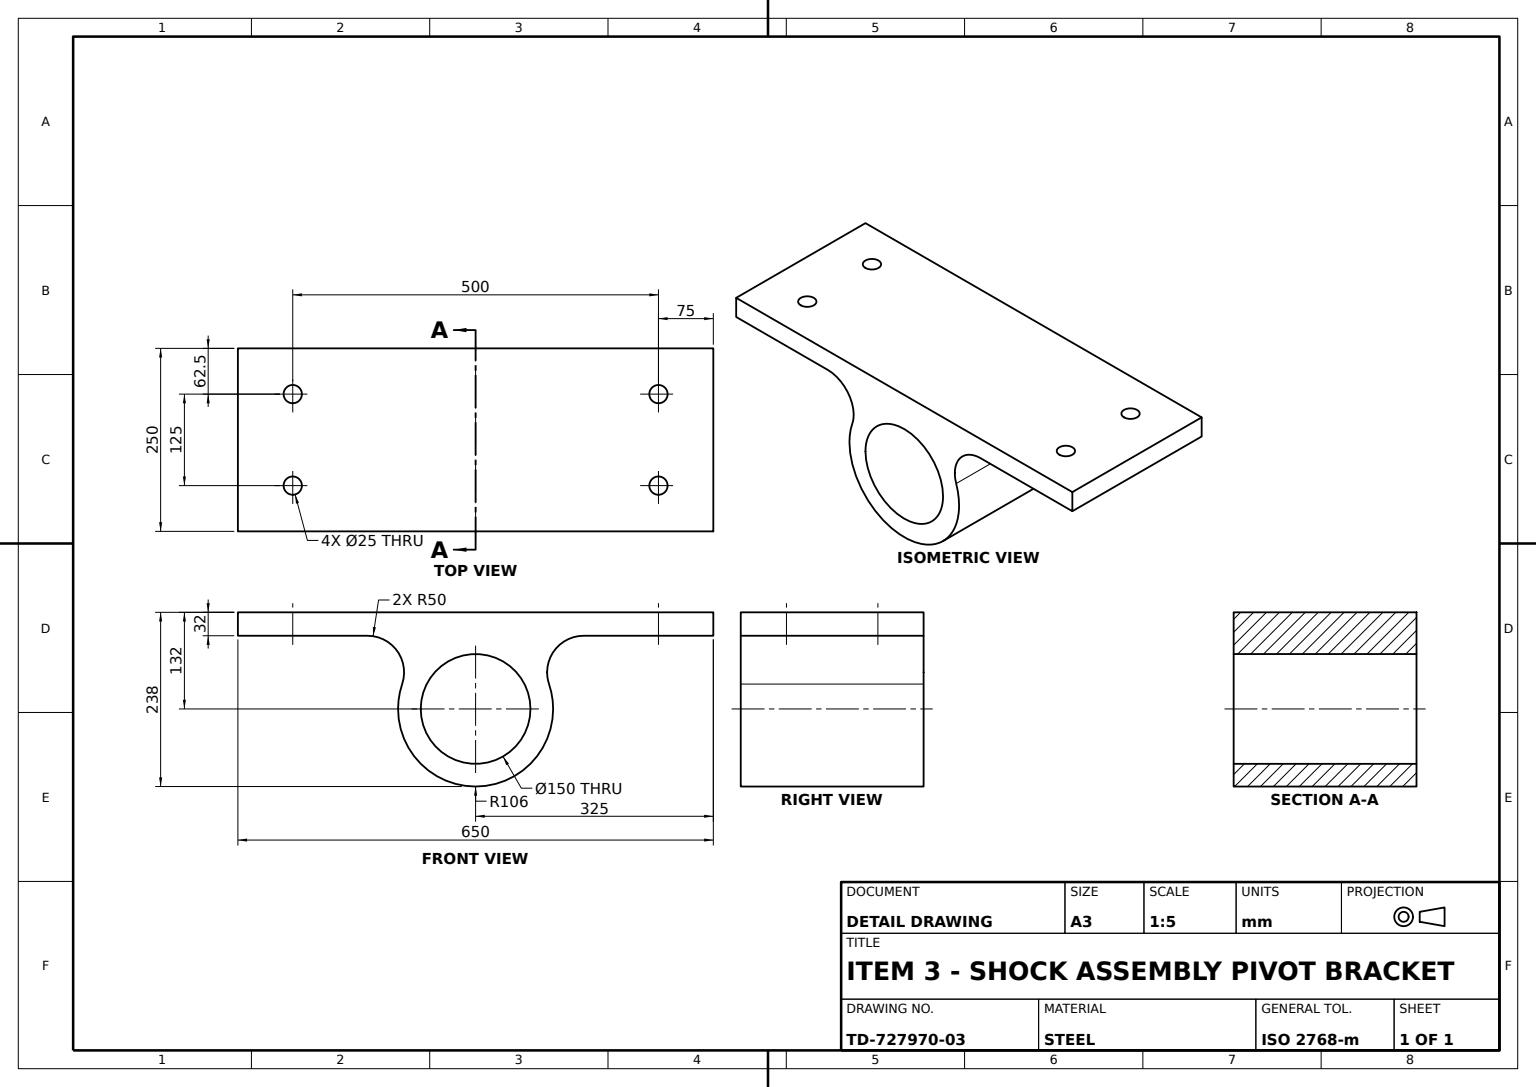
ISO-10303-21;
HEADER;
FILE_DESCRIPTION((''),'2;1');
FILE_NAME('','',(''),(''),'','','');
FILE_SCHEMA(('AUTOMOTIVE_DESIGN'));
ENDSEC;
DATA;
#1=APPLICATION_CONTEXT('');
#2=PRODUCT_CONTEXT('',#1,'mechanical');
#3=PRODUCT('','','',(#2));
#4=PRODUCT_DEFINITION_FORMATION('','',#3);
#5=PRODUCT_DEFINITION_CONTEXT('',#1,'design');
#6=PRODUCT_DEFINITION('','',#4,#5);
#7=PRODUCT_DEFINITION_SHAPE('','',#6);
#8=(LENGTH_UNIT()NAMED_UNIT(*)SI_UNIT(.MILLI.,.METRE.));
#9=(NAMED_UNIT(*)PLANE_ANGLE_UNIT()SI_UNIT($,.RADIAN.));
#10=(NAMED_UNIT(*)SI_UNIT($,.STERADIAN.)SOLID_ANGLE_UNIT());
#11=UNCERTAINTY_MEASURE_WITH_UNIT(LENGTH_MEASURE(1.E-05),#8,'distance_accuracy_value','');
#12=(GEOMETRIC_REPRESENTATION_CONTEXT(3)GLOBAL_UNCERTAINTY_ASSIGNED_CONTEXT((#11))GLOBAL_UNIT_ASSIGNED_CONTEXT((#8,#9,#10))REPRESENTATION_CONTEXT('',''));
#13=CARTESIAN_POINT('',(-250.,132.,75.));
#14=VERTEX_POINT('',#13);
#15=CARTESIAN_POINT('',(-250.,132.,50.));
#16=VERTEX_POINT('',#15);
#17=CARTESIAN_POINT('',(-250.,132.,62.5));
#18=DIRECTION('',(0.,-1.,0.));
#19=DIRECTION('',(0.,0.,-1.));
#20=AXIS2_PLACEMENT_3D('',#17,#18,#19);
#21=CIRCLE('',#20,12.5);
#22=EDGE_CURVE('',#14,#16,#21,.T.);
#23=ORIENTED_EDGE('',*,*,#22,.F.);
#24=CARTESIAN_POINT('',(-250.,100.,75.));
#25=VERTEX_POINT('',#24);
#26=CARTESIAN_POINT('',(-250.,7.,75.));
#27=DIRECTION('',(0.,1.,0.));
#28=VECTOR('',#27,1000.);
#29=LINE('',#26,#28);
#30=EDGE_CURVE('',#25,#14,#29,.T.);
#31=ORIENTED_EDGE('',*,*,#30,.F.);
#32=CARTESIAN_POINT('',(-250.,100.,50.));
#33=VERTEX_POINT('',#32);
#34=CARTESIAN_POINT('',(-250.,100.,62.5));
#35=DIRECTION('',(0.,0.,1.));
#36=AXIS2_PLACEMENT_3D('',#34,#27,#35);
#37=CIRCLE('',#36,12.5);
#38=EDGE_CURVE('',#33,#25,#37,.T.);
#39=ORIENTED_EDGE('',*,*,#38,.F.);
#40=CARTESIAN_POINT('',(-250.,7.,50.));
#41=LINE('',#40,#28);
#42=EDGE_CURVE('',#33,#16,#41,.T.);
#43=ORIENTED_EDGE('',*,*,#42,.T.);
#44=EDGE_LOOP('',(#23,#31,#39,#43));
#45=FACE_OUTER_BOUND('',#44,.T.);
#46=CARTESIAN_POINT('',(-250.,7.,62.5));
#47=AXIS2_PLACEMENT_3D('',#46,#27,#35);
#48=CYLINDRICAL_SURFACE('',#47,12.5);
#49=ADVANCED_FACE('',(#45),#48,.F.);
#50=CARTESIAN_POINT('',(-250.,100.,-75.));
#51=VERTEX_POINT('',#50);
#52=CARTESIAN_POINT('',(-250.,100.,-50.));
#53=VERTEX_POINT('',#52);
#54=CARTESIAN_POINT('',(-250.,100.,-62.5));
#55=AXIS2_PLACEMENT_3D('',#54,#27,#35);
#56=CIRCLE('',#55,12.5);
#57=EDGE_CURVE('',#51,#53,#56,.T.);
#58=ORIENTED_EDGE('',*,*,#57,.T.);
#59=EDGE_CURVE('',#53,#51,#56,.T.);
#60=ORIENTED_EDGE('',*,*,#59,.T.);
#61=EDGE_LOOP('',(#58,#60));
#62=FACE_BOUND('',#61,.T.);
#63=EDGE_CURVE('',#25,#33,#37,.T.);
#64=ORIENTED_EDGE('',*,*,#63,.T.);
#65=ORIENTED_EDGE('',*,*,#38,.T.);
#66=EDGE_LOOP('',(#64,#65));
#67=FACE_BOUND('',#66,.T.);
#68=CARTESIAN_POINT('',(-325.,100.,125.));
#69=VERTEX_POINT('',#68);
#70=CARTESIAN_POINT('',(-147.770092,100.,125.));
#71=VERTEX_POINT('',#70);
#72=DIRECTION('',(1.,0.,0.));
#73=VECTOR('',#72,1000.);
#74=LINE('',#68,#73);
#75=EDGE_CURVE('',#69,#71,#74,.T.);
#76=ORIENTED_EDGE('',*,*,#75,.F.);
#77=CARTESIAN_POINT('',(-325.,100.,-125.));
#78=VERTEX_POINT('',#77);
#79=VECTOR('',#19,1000.);
#80=LINE('',#68,#79);
#81=EDGE_CURVE('',#69,#78,#80,.T.);
#82=ORIENTED_EDGE('',*,*,#81,.T.);
#83=CARTESIAN_POINT('',(-147.770092,100.,-125.));
#84=VERTEX_POINT('',#83);
#85=LINE('',#77,#73);
#86=EDGE_CURVE('',#78,#84,#85,.T.);
#87=ORIENTED_EDGE('',*,*,#86,.T.);
#88=LINE('',#70,#79);
#89=EDGE_CURVE('',#71,#84,#88,.T.);
#90=ORIENTED_EDGE('',*,*,#89,.F.);
#91=EDGE_LOOP('',(#76,#82,#87,#90));
#92=FACE_OUTER_BOUND('',#91,.T.);
#93=AXIS2_PLACEMENT_3D('',#68,#27,#35);
#94=PLANE('',#93);
#95=ADVANCED_FACE('',(#62,#67,#92),#94,.F.);
#96=CARTESIAN_POINT('',(250.,100.,-75.));
#97=VERTEX_POINT('',#96);
#98=CARTESIAN_POINT('',(250.,100.,-50.));
#99=VERTEX_POINT('',#98);
#100=CARTESIAN_POINT('',(250.,100.,-62.5));
#101=AXIS2_PLACEMENT_3D('',#100,#27,#35);
#102=CIRCLE('',#101,12.5);
#103=EDGE_CURVE('',#97,#99,#102,.T.);
#104=ORIENTED_EDGE('',*,*,#103,.T.);
#105=EDGE_CURVE('',#99,#97,#102,.T.);
#106=ORIENTED_EDGE('',*,*,#105,.T.);
#107=EDGE_LOOP('',(#104,#106));
#108=FACE_BOUND('',#107,.T.);
#109=CARTESIAN_POINT('',(325.,100.,125.));
#110=VERTEX_POINT('',#109);
#111=CARTESIAN_POINT('',(325.,100.,-125.));
#112=VERTEX_POINT('',#111);
#113=LINE('',#109,#79);
#114=EDGE_CURVE('',#110,#112,#113,.T.);
#115=ORIENTED_EDGE('',*,*,#114,.F.);
#116=CARTESIAN_POINT('',(147.770092,100.,125.));
#117=VERTEX_POINT('',#116);
#118=LINE('',#116,#73);
#119=EDGE_CURVE('',#117,#110,#118,.T.);
#120=ORIENTED_EDGE('',*,*,#119,.F.);
#121=CARTESIAN_POINT('',(147.770092,100.,-125.));
#122=VERTEX_POINT('',#121);
#123=LINE('',#116,#79);
#124=EDGE_CURVE('',#117,#122,#123,.T.);
#125=ORIENTED_EDGE('',*,*,#124,.T.);
#126=LINE('',#121,#73);
#127=EDGE_CURVE('',#122,#112,#126,.T.);
#128=ORIENTED_EDGE('',*,*,#127,.T.);
#129=EDGE_LOOP('',(#115,#120,#125,#128));
#130=FACE_OUTER_BOUND('',#129,.T.);
#131=CARTESIAN_POINT('',(250.,100.,75.));
#132=VERTEX_POINT('',#131);
#133=CARTESIAN_POINT('',(250.,100.,50.));
#134=VERTEX_POINT('',#133);
#135=CARTESIAN_POINT('',(250.,100.,62.5));
#136=AXIS2_PLACEMENT_3D('',#135,#27,#35);
#137=CIRCLE('',#136,12.5);
#138=EDGE_CURVE('',#132,#134,#137,.T.);
#139=ORIENTED_EDGE('',*,*,#138,.T.);
#140=EDGE_CURVE('',#134,#132,#137,.T.);
#141=ORIENTED_EDGE('',*,*,#140,.T.);
#142=EDGE_LOOP('',(#139,#141));
#143=FACE_BOUND('',#142,.T.);
#144=AXIS2_PLACEMENT_3D('',#116,#27,#35);
#145=PLANE('',#144);
#146=ADVANCED_FACE('',(#108,#130,#143),#145,.F.);
#147=ORIENTED_EDGE('',*,*,#138,.F.);
#148=CARTESIAN_POINT('',(250.,132.,75.));
#149=VERTEX_POINT('',#148);
#150=CARTESIAN_POINT('',(250.,7.,75.));
#151=LINE('',#150,#28);
#152=EDGE_CURVE('',#132,#149,#151,.T.);
#153=ORIENTED_EDGE('',*,*,#152,.T.);
#154=CARTESIAN_POINT('',(250.,132.,50.));
#155=VERTEX_POINT('',#154);
#156=CARTESIAN_POINT('',(250.,132.,62.5));
#157=AXIS2_PLACEMENT_3D('',#156,#18,#19);
#158=CIRCLE('',#157,12.5);
#159=EDGE_CURVE('',#155,#149,#158,.T.);
#160=ORIENTED_EDGE('',*,*,#159,.F.);
#161=CARTESIAN_POINT('',(250.,7.,50.));
#162=LINE('',#161,#28);
#163=EDGE_CURVE('',#134,#155,#162,.T.);
#164=ORIENTED_EDGE('',*,*,#163,.F.);
#165=EDGE_LOOP('',(#147,#153,#160,#164));
#166=FACE_OUTER_BOUND('',#165,.T.);
#167=CARTESIAN_POINT('',(250.,7.,62.5));
#168=AXIS2_PLACEMENT_3D('',#167,#27,#35);
#169=CYLINDRICAL_SURFACE('',#168,12.5);
#170=ADVANCED_FACE('',(#166),#169,.F.);
#171=CARTESIAN_POINT('',(75.,0.,125.));
#172=VERTEX_POINT('',#171);
#173=CARTESIAN_POINT('',(75.,0.,-125.));
#174=VERTEX_POINT('',#173);
#175=LINE('',#171,#79);
#176=EDGE_CURVE('',#172,#174,#175,.T.);
#177=ORIENTED_EDGE('',*,*,#176,.F.);
#178=CARTESIAN_POINT('',(-75.,0.,125.));
#179=VERTEX_POINT('',#178);
#180=CARTESIAN_POINT('',(0.,0.,125.));
#181=AXIS2_PLACEMENT_3D('',#180,#35,#72);
#182=CIRCLE('',#181,75.);
#183=EDGE_CURVE('',#172,#179,#182,.T.);
#184=ORIENTED_EDGE('',*,*,#183,.T.);
#185=CARTESIAN_POINT('',(-75.,0.,-125.));
#186=VERTEX_POINT('',#185);
#187=LINE('',#178,#79);
#188=EDGE_CURVE('',#179,#186,#187,.T.);
#189=ORIENTED_EDGE('',*,*,#188,.T.);
#190=CARTESIAN_POINT('',(0.,0.,-125.));
#191=AXIS2_PLACEMENT_3D('',#190,#35,#72);
#192=CIRCLE('',#191,75.);
#193=EDGE_CURVE('',#174,#186,#192,.T.);
#194=ORIENTED_EDGE('',*,*,#193,.F.);
#195=EDGE_LOOP('',(#177,#184,#189,#194));
#196=FACE_OUTER_BOUND('',#195,.T.);
#197=DIRECTION('',(-1.,0.,0.));
#198=AXIS2_PLACEMENT_3D('',#180,#19,#197);
#199=CYLINDRICAL_SURFACE('',#198,75.);
#200=ADVANCED_FACE('',(#196),#199,.F.);
#201=ORIENTED_EDGE('',*,*,#183,.F.);
#202=EDGE_CURVE('',#179,#172,#182,.T.);
#203=ORIENTED_EDGE('',*,*,#202,.F.);
#204=EDGE_LOOP('',(#201,#203));
#205=FACE_BOUND('',#204,.T.);
#206=CARTESIAN_POINT('',(106.,0.,125.));
#207=VERTEX_POINT('',#206);
#208=CARTESIAN_POINT('',(100.407883,33.974359,125.));
#209=VERTEX_POINT('',#208);
#210=CIRCLE('',#181,106.);
#211=EDGE_CURVE('',#207,#209,#210,.T.);
#212=ORIENTED_EDGE('',*,*,#211,.T.);
#213=CARTESIAN_POINT('',(97.770092,50.,125.));
#214=VERTEX_POINT('',#213);
#215=CARTESIAN_POINT('',(147.770092,50.,125.));
#216=AXIS2_PLACEMENT_3D('',#215,#19,#72);
#217=CIRCLE('',#216,50.);
#218=EDGE_CURVE('',#209,#214,#217,.T.);
#219=ORIENTED_EDGE('',*,*,#218,.T.);
#220=EDGE_CURVE('',#214,#117,#217,.T.);
#221=ORIENTED_EDGE('',*,*,#220,.T.);
#222=ORIENTED_EDGE('',*,*,#119,.T.);
#223=CARTESIAN_POINT('',(325.,132.,125.));
#224=VERTEX_POINT('',#223);
#225=LINE('',#223,#28);
#226=EDGE_CURVE('',#110,#224,#225,.T.);
#227=ORIENTED_EDGE('',*,*,#226,.T.);
#228=CARTESIAN_POINT('',(-325.,132.,125.));
#229=VERTEX_POINT('',#228);
#230=VECTOR('',#197,1000.);
#231=LINE('',#228,#230);
#232=EDGE_CURVE('',#224,#229,#231,.T.);
#233=ORIENTED_EDGE('',*,*,#232,.T.);
#234=VECTOR('',#18,1000.);
#235=LINE('',#228,#234);
#236=EDGE_CURVE('',#229,#69,#235,.T.);
#237=ORIENTED_EDGE('',*,*,#236,.T.);
#238=ORIENTED_EDGE('',*,*,#75,.T.);
#239=CARTESIAN_POINT('',(-100.407883,33.974359,125.));
#240=VERTEX_POINT('',#239);
#241=CARTESIAN_POINT('',(-147.770092,50.,125.));
#242=AXIS2_PLACEMENT_3D('',#241,#19,#72);
#243=CIRCLE('',#242,50.);
#244=EDGE_CURVE('',#71,#240,#243,.T.);
#245=ORIENTED_EDGE('',*,*,#244,.T.);
#246=CARTESIAN_POINT('',(-106.,0.,125.));
#247=VERTEX_POINT('',#246);
#248=EDGE_CURVE('',#240,#247,#210,.T.);
#249=ORIENTED_EDGE('',*,*,#248,.T.);
#250=EDGE_CURVE('',#247,#207,#210,.T.);
#251=ORIENTED_EDGE('',*,*,#250,.T.);
#252=EDGE_LOOP('',(#212,#219,#221,#222,#227,#233,#237,#238,#245,#249,#251));
#253=FACE_OUTER_BOUND('',#252,.T.);
#254=AXIS2_PLACEMENT_3D('',#215,#35,#72);
#255=PLANE('',#254);
#256=ADVANCED_FACE('',(#205,#253),#255,.T.);
#257=CARTESIAN_POINT('',(250.,132.,-50.));
#258=VERTEX_POINT('',#257);
#259=CARTESIAN_POINT('',(250.,7.,-50.));
#260=LINE('',#259,#28);
#261=EDGE_CURVE('',#99,#258,#260,.T.);
#262=ORIENTED_EDGE('',*,*,#261,.T.);
#263=CARTESIAN_POINT('',(250.,132.,-75.));
#264=VERTEX_POINT('',#263);
#265=CARTESIAN_POINT('',(250.,132.,-62.5));
#266=AXIS2_PLACEMENT_3D('',#265,#18,#19);
#267=CIRCLE('',#266,12.5);
#268=EDGE_CURVE('',#264,#258,#267,.T.);
#269=ORIENTED_EDGE('',*,*,#268,.F.);
#270=CARTESIAN_POINT('',(250.,7.,-75.));
#271=LINE('',#270,#28);
#272=EDGE_CURVE('',#97,#264,#271,.T.);
#273=ORIENTED_EDGE('',*,*,#272,.F.);
#274=ORIENTED_EDGE('',*,*,#105,.F.);
#275=EDGE_LOOP('',(#262,#269,#273,#274));
#276=FACE_OUTER_BOUND('',#275,.T.);
#277=CARTESIAN_POINT('',(250.,7.,-62.5));
#278=AXIS2_PLACEMENT_3D('',#277,#27,#35);
#279=CYLINDRICAL_SURFACE('',#278,12.5);
#280=ADVANCED_FACE('',(#276),#279,.F.);
#281=ORIENTED_EDGE('',*,*,#57,.F.);
#282=CARTESIAN_POINT('',(-250.,132.,-75.));
#283=VERTEX_POINT('',#282);
#284=CARTESIAN_POINT('',(-250.,7.,-75.));
#285=LINE('',#284,#28);
#286=EDGE_CURVE('',#51,#283,#285,.T.);
#287=ORIENTED_EDGE('',*,*,#286,.T.);
#288=CARTESIAN_POINT('',(-250.,132.,-50.));
#289=VERTEX_POINT('',#288);
#290=CARTESIAN_POINT('',(-250.,132.,-62.5));
#291=AXIS2_PLACEMENT_3D('',#290,#18,#19);
#292=CIRCLE('',#291,12.5);
#293=EDGE_CURVE('',#289,#283,#292,.T.);
#294=ORIENTED_EDGE('',*,*,#293,.F.);
#295=CARTESIAN_POINT('',(-250.,7.,-50.));
#296=LINE('',#295,#28);
#297=EDGE_CURVE('',#53,#289,#296,.T.);
#298=ORIENTED_EDGE('',*,*,#297,.F.);
#299=EDGE_LOOP('',(#281,#287,#294,#298));
#300=FACE_OUTER_BOUND('',#299,.T.);
#301=CARTESIAN_POINT('',(-250.,7.,-62.5));
#302=AXIS2_PLACEMENT_3D('',#301,#27,#35);
#303=CYLINDRICAL_SURFACE('',#302,12.5);
#304=ADVANCED_FACE('',(#300),#303,.F.);
#305=CARTESIAN_POINT('',(-100.407883,33.974359,-125.));
#306=VERTEX_POINT('',#305);
#307=CARTESIAN_POINT('',(-147.770092,50.,-125.));
#308=AXIS2_PLACEMENT_3D('',#307,#19,#72);
#309=CIRCLE('',#308,50.);
#310=EDGE_CURVE('',#84,#306,#309,.T.);
#311=ORIENTED_EDGE('',*,*,#310,.T.);
#312=LINE('',#239,#79);
#313=EDGE_CURVE('',#240,#306,#312,.T.);
#314=ORIENTED_EDGE('',*,*,#313,.F.);
#315=ORIENTED_EDGE('',*,*,#244,.F.);
#316=ORIENTED_EDGE('',*,*,#89,.T.);
#317=EDGE_LOOP('',(#311,#314,#315,#316));
#318=FACE_OUTER_BOUND('',#317,.T.);
#319=AXIS2_PLACEMENT_3D('',#241,#19,#197);
#320=CYLINDRICAL_SURFACE('',#319,50.);
#321=ADVANCED_FACE('',(#318),#320,.F.);
#322=ORIENTED_EDGE('',*,*,#152,.F.);
#323=ORIENTED_EDGE('',*,*,#140,.F.);
#324=ORIENTED_EDGE('',*,*,#163,.T.);
#325=EDGE_CURVE('',#149,#155,#158,.T.);
#326=ORIENTED_EDGE('',*,*,#325,.F.);
#327=EDGE_LOOP('',(#322,#323,#324,#326));
#328=FACE_OUTER_BOUND('',#327,.T.);
#329=ADVANCED_FACE('',(#328),#169,.F.);
#330=ORIENTED_EDGE('',*,*,#236,.F.);
#331=CARTESIAN_POINT('',(-325.,132.,-125.));
#332=VERTEX_POINT('',#331);
#333=LINE('',#228,#79);
#334=EDGE_CURVE('',#229,#332,#333,.T.);
#335=ORIENTED_EDGE('',*,*,#334,.T.);
#336=LINE('',#331,#234);
#337=EDGE_CURVE('',#332,#78,#336,.T.);
#338=ORIENTED_EDGE('',*,*,#337,.T.);
#339=ORIENTED_EDGE('',*,*,#81,.F.);
#340=EDGE_LOOP('',(#330,#335,#338,#339));
#341=FACE_OUTER_BOUND('',#340,.T.);
#342=AXIS2_PLACEMENT_3D('',#228,#72,#19);
#343=PLANE('',#342);
#344=ADVANCED_FACE('',(#341),#343,.F.);
#345=CARTESIAN_POINT('',(325.,132.,-125.));
#346=VERTEX_POINT('',#345);
#347=LINE('',#223,#79);
#348=EDGE_CURVE('',#224,#346,#347,.T.);
#349=ORIENTED_EDGE('',*,*,#348,.F.);
#350=ORIENTED_EDGE('',*,*,#226,.F.);
#351=ORIENTED_EDGE('',*,*,#114,.T.);
#352=LINE('',#345,#28);
#353=EDGE_CURVE('',#112,#346,#352,.T.);
#354=ORIENTED_EDGE('',*,*,#353,.T.);
#355=EDGE_LOOP('',(#349,#350,#351,#354));
#356=FACE_OUTER_BOUND('',#355,.T.);
#357=AXIS2_PLACEMENT_3D('',#223,#197,#18);
#358=PLANE('',#357);
#359=ADVANCED_FACE('',(#356),#358,.F.);
#360=ORIENTED_EDGE('',*,*,#313,.T.);
#361=CARTESIAN_POINT('',(-106.,0.,-125.));
#362=VERTEX_POINT('',#361);
#363=CIRCLE('',#191,106.);
#364=EDGE_CURVE('',#306,#362,#363,.T.);
#365=ORIENTED_EDGE('',*,*,#364,.T.);
#366=LINE('',#246,#79);
#367=EDGE_CURVE('',#247,#362,#366,.T.);
#368=ORIENTED_EDGE('',*,*,#367,.F.);
#369=ORIENTED_EDGE('',*,*,#248,.F.);
#370=EDGE_LOOP('',(#360,#365,#368,#369));
#371=FACE_OUTER_BOUND('',#370,.T.);
#372=CYLINDRICAL_SURFACE('',#198,106.);
#373=ADVANCED_FACE('',(#371),#372,.T.);
#374=EDGE_CURVE('',#283,#289,#292,.T.);
#375=ORIENTED_EDGE('',*,*,#374,.F.);
#376=ORIENTED_EDGE('',*,*,#286,.F.);
#377=ORIENTED_EDGE('',*,*,#59,.F.);
#378=ORIENTED_EDGE('',*,*,#297,.T.);
#379=EDGE_LOOP('',(#375,#376,#377,#378));
#380=FACE_OUTER_BOUND('',#379,.T.);
#381=ADVANCED_FACE('',(#380),#303,.F.);
#382=CARTESIAN_POINT('',(106.,0.,-125.));
#383=VERTEX_POINT('',#382);
#384=LINE('',#206,#79);
#385=EDGE_CURVE('',#207,#383,#384,.T.);
#386=ORIENTED_EDGE('',*,*,#385,.F.);
#387=ORIENTED_EDGE('',*,*,#250,.F.);
#388=ORIENTED_EDGE('',*,*,#367,.T.);
#389=EDGE_CURVE('',#362,#383,#363,.T.);
#390=ORIENTED_EDGE('',*,*,#389,.T.);
#391=EDGE_LOOP('',(#386,#387,#388,#390));
#392=FACE_OUTER_BOUND('',#391,.T.);
#393=ADVANCED_FACE('',(#392),#372,.T.);
#394=LINE('',#331,#230);
#395=EDGE_CURVE('',#346,#332,#394,.T.);
#396=ORIENTED_EDGE('',*,*,#395,.T.);
#397=ORIENTED_EDGE('',*,*,#334,.F.);
#398=ORIENTED_EDGE('',*,*,#232,.F.);
#399=ORIENTED_EDGE('',*,*,#348,.T.);
#400=EDGE_LOOP('',(#396,#397,#398,#399));
#401=FACE_OUTER_BOUND('',#400,.T.);
#402=ORIENTED_EDGE('',*,*,#268,.T.);
#403=EDGE_CURVE('',#258,#264,#267,.T.);
#404=ORIENTED_EDGE('',*,*,#403,.T.);
#405=EDGE_LOOP('',(#402,#404));
#406=FACE_BOUND('',#405,.T.);
#407=ORIENTED_EDGE('',*,*,#159,.T.);
#408=ORIENTED_EDGE('',*,*,#325,.T.);
#409=EDGE_LOOP('',(#407,#408));
#410=FACE_BOUND('',#409,.T.);
#411=ORIENTED_EDGE('',*,*,#22,.T.);
#412=EDGE_CURVE('',#16,#14,#21,.T.);
#413=ORIENTED_EDGE('',*,*,#412,.T.);
#414=EDGE_LOOP('',(#411,#413));
#415=FACE_BOUND('',#414,.T.);
#416=ORIENTED_EDGE('',*,*,#293,.T.);
#417=ORIENTED_EDGE('',*,*,#374,.T.);
#418=EDGE_LOOP('',(#416,#417));
#419=FACE_BOUND('',#418,.T.);
#420=AXIS2_PLACEMENT_3D('',#228,#18,#19);
#421=PLANE('',#420);
#422=ADVANCED_FACE('',(#401,#406,#410,#415,#419),#421,.F.);
#423=CARTESIAN_POINT('',(97.770092,50.,-125.));
#424=VERTEX_POINT('',#423);
#425=LINE('',#213,#79);
#426=EDGE_CURVE('',#214,#424,#425,.T.);
#427=ORIENTED_EDGE('',*,*,#426,.T.);
#428=CARTESIAN_POINT('',(147.770092,50.,-125.));
#429=AXIS2_PLACEMENT_3D('',#428,#19,#72);
#430=CIRCLE('',#429,50.);
#431=EDGE_CURVE('',#424,#122,#430,.T.);
#432=ORIENTED_EDGE('',*,*,#431,.T.);
#433=ORIENTED_EDGE('',*,*,#124,.F.);
#434=ORIENTED_EDGE('',*,*,#220,.F.);
#435=EDGE_LOOP('',(#427,#432,#433,#434));
#436=FACE_OUTER_BOUND('',#435,.T.);
#437=AXIS2_PLACEMENT_3D('',#215,#19,#197);
#438=CYLINDRICAL_SURFACE('',#437,50.);
#439=ADVANCED_FACE('',(#436),#438,.F.);
#440=EDGE_CURVE('',#186,#174,#192,.T.);
#441=ORIENTED_EDGE('',*,*,#440,.T.);
#442=ORIENTED_EDGE('',*,*,#193,.T.);
#443=EDGE_LOOP('',(#441,#442));
#444=FACE_BOUND('',#443,.T.);
#445=ORIENTED_EDGE('',*,*,#431,.F.);
#446=CARTESIAN_POINT('',(100.407883,33.974359,-125.));
#447=VERTEX_POINT('',#446);
#448=EDGE_CURVE('',#447,#424,#430,.T.);
#449=ORIENTED_EDGE('',*,*,#448,.F.);
#450=EDGE_CURVE('',#383,#447,#363,.T.);
#451=ORIENTED_EDGE('',*,*,#450,.F.);
#452=ORIENTED_EDGE('',*,*,#389,.F.);
#453=ORIENTED_EDGE('',*,*,#364,.F.);
#454=ORIENTED_EDGE('',*,*,#310,.F.);
#455=ORIENTED_EDGE('',*,*,#86,.F.);
#456=ORIENTED_EDGE('',*,*,#337,.F.);
#457=ORIENTED_EDGE('',*,*,#395,.F.);
#458=ORIENTED_EDGE('',*,*,#353,.F.);
#459=ORIENTED_EDGE('',*,*,#127,.F.);
#460=EDGE_LOOP('',(#445,#449,#451,#452,#453,#454,#455,#456,#457,#458,#459));
#461=FACE_OUTER_BOUND('',#460,.T.);
#462=AXIS2_PLACEMENT_3D('',#428,#35,#72);
#463=PLANE('',#462);
#464=ADVANCED_FACE('',(#444,#461),#463,.F.);
#465=ORIENTED_EDGE('',*,*,#103,.F.);
#466=ORIENTED_EDGE('',*,*,#272,.T.);
#467=ORIENTED_EDGE('',*,*,#403,.F.);
#468=ORIENTED_EDGE('',*,*,#261,.F.);
#469=EDGE_LOOP('',(#465,#466,#467,#468));
#470=FACE_OUTER_BOUND('',#469,.T.);
#471=ADVANCED_FACE('',(#470),#279,.F.);
#472=ORIENTED_EDGE('',*,*,#440,.F.);
#473=ORIENTED_EDGE('',*,*,#188,.F.);
#474=ORIENTED_EDGE('',*,*,#202,.T.);
#475=ORIENTED_EDGE('',*,*,#176,.T.);
#476=EDGE_LOOP('',(#472,#473,#474,#475));
#477=FACE_OUTER_BOUND('',#476,.T.);
#478=ADVANCED_FACE('',(#477),#199,.F.);
#479=ORIENTED_EDGE('',*,*,#448,.T.);
#480=ORIENTED_EDGE('',*,*,#426,.F.);
#481=ORIENTED_EDGE('',*,*,#218,.F.);
#482=LINE('',#208,#79);
#483=EDGE_CURVE('',#209,#447,#482,.T.);
#484=ORIENTED_EDGE('',*,*,#483,.T.);
#485=EDGE_LOOP('',(#479,#480,#481,#484));
#486=FACE_OUTER_BOUND('',#485,.T.);
#487=ADVANCED_FACE('',(#486),#438,.F.);
#488=ORIENTED_EDGE('',*,*,#450,.T.);
#489=ORIENTED_EDGE('',*,*,#483,.F.);
#490=ORIENTED_EDGE('',*,*,#211,.F.);
#491=ORIENTED_EDGE('',*,*,#385,.T.);
#492=EDGE_LOOP('',(#488,#489,#490,#491));
#493=FACE_OUTER_BOUND('',#492,.T.);
#494=ADVANCED_FACE('',(#493),#372,.T.);
#495=ORIENTED_EDGE('',*,*,#30,.T.);
#496=ORIENTED_EDGE('',*,*,#412,.F.);
#497=ORIENTED_EDGE('',*,*,#42,.F.);
#498=ORIENTED_EDGE('',*,*,#63,.F.);
#499=EDGE_LOOP('',(#495,#496,#497,#498));
#500=FACE_OUTER_BOUND('',#499,.T.);
#501=ADVANCED_FACE('',(#500),#48,.F.);
#502=CLOSED_SHELL('',(#49,#95,#146,#170,#200,#256,#280,#304,#321,#329,#344,#359,#373,#381,#393,#422,#439,#464,#471,#478,#487,#494,#501));
#503=MANIFOLD_SOLID_BREP('',#502);
#504=ADVANCED_BREP_SHAPE_REPRESENTATION('',(#503),#12);
#505=SHAPE_DEFINITION_REPRESENTATION(#7,#504);
ENDSEC;
END-ISO-10303-21;
